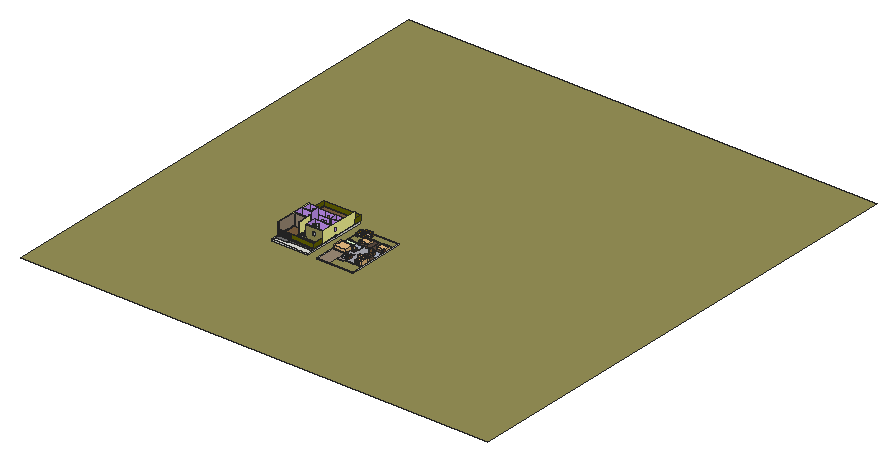
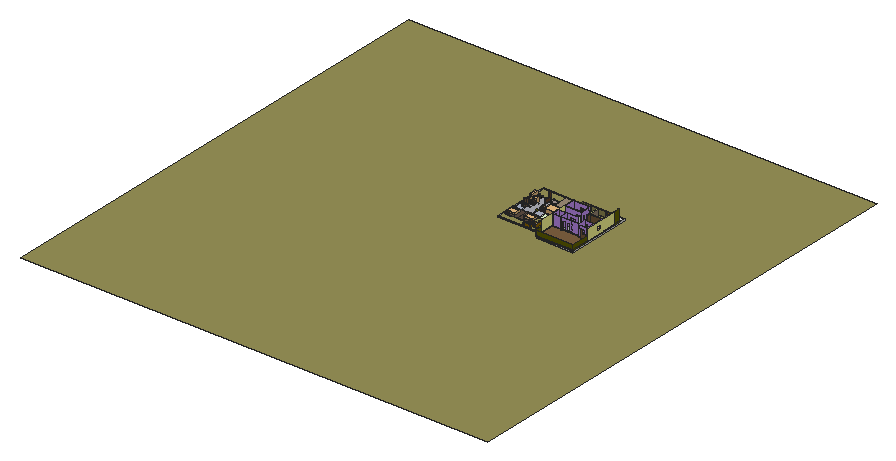
# SketchUp Ruby script. Lengths in inches.
U = 1.inch
M = Sketchup.active_model
def pt(a) = Geom::Point3d.new(a.map { |v| v * U })
def face(e, loops, mat)
  f = e.add_face(loops[0].map { |a| pt(a) })
  loops[1..].each { |l| e.add_face(l.map { |a| pt(a) }).erase! }
  f.material = f.back_material = mat if mat
  f
end
# faces: each face lists its corners as indices into pts; further lists are holes
def faces(e, pts, list, mat = nil) = list.each { |f| face(e, (f[0].is_a?(Array) ? f : [f]).map { |l| l.map { |i| pts[i] } }, mat) }
# xy, xz, yz: faces in a plane at the given z, y or x. An outline is a flat list of corners, or four numbers for a rectangle; further outlines are holes
def ring(l) = l.size == 4 ? [[l[0], l[1]], [l[2], l[1]], [l[2], l[3]], [l[0], l[3]]] : l.each_slice(2).to_a
def flat(e, list, mat, &to3) = list.each { |f| face(e, (f[0].is_a?(Array) ? f : [f]).map { |l| ring(l).map { |u, v| to3.(u, v) } }, mat) }
def xy(e, z, list, mat = nil) = flat(e, list, mat) { |x, y| [x, y, z] }
def xz(e, y, list, mat = nil) = flat(e, list, mat) { |x, z| [x, y, z] }
def yz(e, x, list, mat = nil) = flat(e, list, mat) { |y, z| [x, y, z] }
def lines(e, pts, list) = list.each { |a, b| e.add_line(pt(pts[a]), pt(pts[b])) }
# prism: a flat outline (further loops are holes) pulled along v
def prism(e, loops, v, mat = nil)
  f = face(e, loops, mat); d = Geom::Vector3d.new(v.map { |x| x * U })
  f.pushpull(f.normal.samedirection?(d) ? d.length : -d.length)
end
def box(e, o, s, mat = nil) = prism(e, [[o, [o[0] + s[0], o[1], o[2]], [o[0] + s[0], o[1] + s[1], o[2]], [o[0], o[1] + s[1], o[2]]]], [0, 0, s[2]], mat)
def at(x, y, z, deg = 0) = Geom::Transformation.translation(pt([x, y, z])) * Geom::Transformation.rotation(ORIGIN, Z_AXIS, deg.degrees)
def axes(o, x, y, z) = Geom::Transformation.new([*x, 0, *y, 0, *z, 0, *pt(o).to_a, 1])
def part(name) = M.definitions.add(name)
# library, detail: a bought-in or finely detailed component or shape, given as its bounding box
def library(name, o, s) = part(name).tap { |d| box(d.entities, o, s) }
def detail(e, o, s) = box(e.add_group.entities, o, s)
def put(e, d, t, mat = nil) = e.add_instance(d, t).tap { |i| i.material = mat if mat }
def group(e, t, mat = nil) = e.add_group.tap { |g| g.transformation = t; g.material = mat if mat }.entities
root = M.entities
M.materials.add("C01_Vanilla_Cream").color = [255, 230, 206]
M.materials.add("D07_Ochre_Flame").color = [153, 107, 0]
M.materials.add("E01_Mint_Frost").color = [255, 255, 204]
M.materials.add("E02_Pale_Lime").color = [255, 255, 153]
M.materials.add("E08_Lime_Depth").color = [102, 102, 0]
M.materials.add("Glass_Sky Reflection_01").color = [126, 138, 183]
M.materials["Glass_Sky Reflection_01"].alpha = 0.25
M.materials.add("J02_Lavender_Veil").color = [204, 153, 255]
M.materials.add("M05_Graphite_Haze").color = [114, 114, 114]
M.materials.add("M09_Shadow_Night").color = [0, 0, 0]
M.materials.add("Marble_01_1K").color = [230, 255, 211]
M.materials.add("Marble_03_1K").color = [175, 182, 201]
M.materials.add("Marble_06_1K").color = [165, 150, 147]
M.materials.add("Marble_07_1K").color = [36, 34, 36]
M.materials.add("Marble_20_1K").color = [172, 173, 182]
M.materials.add("Metal_06_1K").color = [238, 236, 231]
M.materials.add("Plaster_02_1K").color = [157, 140, 119]
M.materials.add("Plywood_01_1K").color = [125, 96, 64]
M.materials.add("Soil_04_1K").color = [152, 146, 88]
M.materials.add("Wood_Floor_01_1K").color = [146, 111, 76]
M.materials.add("Wood_Floor_12_1K").color = [92, 75, 65]
M.materials.add("Wood_Veneer_15_1K").color = [103, 69, 45]
c1 = library("Group\#68",[0,0,0],[137.375,104.9375,36.125])
c2 = library("Group\#24",[0,0,0],[4.375,4.375,0.1875])
c3 = part("Group\#9")
box(c3.entities,[0,0,0],[0.75,3.75,0.1875],"Metal_06_1K")
c4 = part("Group\#2")
xy(c4.entities,0,[[0,-16.81,18.0625,0],[0,0,18.0625,55.25]],"Wood_Veneer_15_1K")
xy(c4.entities,36,[[0,0,18.0625,55.25]],"Wood_Veneer_15_1K")
xy(c4.entities,84,[[0,-16.81,18.0625,0]],"Wood_Veneer_15_1K")
xz(c4.entities,-16.81,[[0,0,18.0625,84]],"Wood_Veneer_15_1K")
xz(c4.entities,0,[[0,0,18.0625,36],[0,36,18.0625,84]],"Wood_Veneer_15_1K")
xz(c4.entities,55.25,[[0,0,18.0625,36]],"Wood_Veneer_15_1K")
yz(c4.entities,0,[[-16.81,0,0,84],[0,0,55.25,36]],"Wood_Veneer_15_1K")
yz(c4.entities,18.0625,[[[-16.81,0,0,84],[-14.81,2,-2,82]],[0,0,27.625,27.91],[27.625,0,55.25,27.91],[-14.81,2,-2,35],[0,27.91,55.25,36],
  [-14.81,35,-2,36],[-14.81,36,-2,50.3125],[-14.81,50.3125,-2,51.3125],[-14.81,51.3125,-2,65.85],[-14.81,65.85,-2,66.85],
  [-14.81,66.85,-2,82]],"Wood_Veneer_15_1K")
g1 = group(c4.entities,at(18.0625,23.18,16.77))
box(g1,[0,0,0],[0.2,1.5,6.25],"Metal_06_1K")
g2 = group(c4.entities,at(18.0625,29.74,16.77))
box(g2,[0,0,0],[0.2,1.5,6.25],"Metal_06_1K")
put(c4.entities,c3,axes([18.0625,-4.49,72.03],[0,1,0],[0,0,1],[1,0,0]))
put(c4.entities,c3,axes([18.0625,-4.49,57.4],[0,1,0],[0,0,1],[1,0,0]))
put(c4.entities,c3,axes([18.0625,-4.49,42.9],[0,1,0],[0,0,1],[1,0,0]))
put(c4.entities,c3,axes([18.0625,-4.49,20.71],[0,1,0],[0,0,1],[1,0,0]))
c5 = part("Group\#41")
xy(c5.entities,0,[[[0,0,32.5625,34],[3.65,3.65,28.91,30.35]]],"D07_Ochre_Flame")
xy(c5.entities,18.3125,[[[0,0,32.5625,34],[3.65,3.65,28.91,30.35]]],"D07_Ochre_Flame")
xy(c5.entities,18.3125,[[3.65,3.65,28.91,30.35]],"Plaster_02_1K")
xz(c5.entities,0,[[0,0,32.5625,18.3125]],"D07_Ochre_Flame")
xz(c5.entities,3.65,[[3.65,0,28.91,18.3125]],"D07_Ochre_Flame")
xz(c5.entities,30.35,[[3.65,0,28.91,18.3125]],"D07_Ochre_Flame")
xz(c5.entities,34,[[0,0,32.5625,18.3125]],"D07_Ochre_Flame")
yz(c5.entities,0,[[0,0,34,18.3125]],"D07_Ochre_Flame")
yz(c5.entities,3.65,[[3.65,0,30.35,18.3125]],"D07_Ochre_Flame")
yz(c5.entities,28.91,[[3.65,0,30.35,18.3125]],"D07_Ochre_Flame")
yz(c5.entities,32.5625,[[0,0,34,18.3125]],"D07_Ochre_Flame")
c6 = library("Group\#27",[0,0,0],[94.3125,62.5,20])
c7 = part("Group\#17")
box(c7.entities,[0,0,0],[4,4,24])
c8 = part("Group\#16")
box(c8.entities,[0,0,0],[4,4,24])
c9 = part("Group\#29")
box(c9.entities,[0,0,0],[20.5,20.5,18],"Wood_Veneer_15_1K")
c10 = part("Group\#12")
detail(c10.entities,[-3,0,0],[54,27,43.625])
c11 = part("Group\#11")
detail(c11.entities,[0,0,0],[24,24,25.375])
c12 = part("Group\#10")
detail(c12.entities,[0,-4,0],[28,80,43.625])
c13 = part("Group\#14")
box(c13.entities,[0,0,0],[4,4,24])
c14 = part("Group\#15")
box(c14.entities,[0,0,0],[4,4,24])
c15 = part("Group\#38")
xy(c15.entities,0,[[67.3125,0,69.625,27.1875],[-2.33,24.1875,67.3125,27.1875]],"D07_Ochre_Flame")
xy(c15.entities,18.3125,[[0,0,22.82,24.1875],[22.82,0,45.07,24.1875],[45.07,0,67.3125,24.1875]],"C01_Vanilla_Cream")
xy(c15.entities,24.5625,[[67.3125,0,69.625,27.1875]],"D07_Ochre_Flame")
xy(c15.entities,28.6875,[[-2.33,0,0,24.1875]],"D07_Ochre_Flame")
xy(c15.entities,33.375,[[-2.33,24.1875,67.3125,27.1875]],"D07_Ochre_Flame")
xz(c15.entities,0,[[0,0,22.82,18.3125],[22.82,0,45.07,18.3125],[45.07,0,67.3125,18.3125]],"C01_Vanilla_Cream")
xz(c15.entities,0,[[-2.33,0,0,28.6875],[67.3125,0,69.625,24.5625]],"D07_Ochre_Flame")
xz(c15.entities,24.1875,[[-2.33,0,67.3125,0,67.3125,18.3125,0,18.3125,0,28.6875,-2.33,28.6875],[0,18.3125,22.82,33.375],[22.82,18.3125,45.07,33.375],[45.07,18.3125,67.3125,33.375],[-2.33,28.6875,0,33.375]],"D07_Ochre_Flame")
xz(c15.entities,27.1875,[[-2.33,0,67.3125,33.375],[67.3125,0,69.625,24.5625]],"D07_Ochre_Flame")
yz(c15.entities,-2.33,[[0,0,24.1875,28.6875],[24.1875,0,27.1875,33.375]],"D07_Ochre_Flame")
yz(c15.entities,0,[[0,18.3125,24.1875,28.6875]],"D07_Ochre_Flame")
yz(c15.entities,67.3125,[[0,0,24.1875,18.3125],[0,18.3125,24.1875,24.5625]],"C01_Vanilla_Cream")
yz(c15.entities,67.3125,[[24.1875,0,27.1875,24.5625],[24.1875,24.5625,27.1875,33.375]],"D07_Ochre_Flame")
yz(c15.entities,69.625,[[0,0,27.1875,24.5625]],"D07_Ochre_Flame")
c16 = part("Group\#43")
box(c16.entities,[0,0,0],[1,4.5625,0.25],"Metal_06_1K")
c17 = part("Group\#42")
xy(c17.entities,0,[[0,-1.93,40.35,0],[0,0,40.35,21.25]],"Plywood_01_1K")
xy(c17.entities,25.125,[[0,0,40.35,21.25]],"Marble_07_1K")
xy(c17.entities,25.1875,[[20.85,8.75,21.39,8.86,21.89,9.11,22.3,9.47,22.61,9.94,22.79,10.46,22.82,11.01,22.71,11.56,22.47,12.06,22.1,12.47,21.64,12.78,21.11,12.96,20.56,12.99,20.01,12.88,19.52,12.63,19.1,12.27,18.79,11.81,18.62,11.28,18.58,10.73,18.69,10.18,18.9375,9.69,19.31,9.27,19.77,8.96,20.29,8.79]],"M09_Shadow_Night")
xy(c17.entities,25.1875,[[[8.8,4,31.8,17.68],[20.85,8.75,20.29,8.79,19.77,8.96,19.31,9.27,18.9375,9.69,18.69,10.18,18.58,10.73,18.62,11.28,18.79,11.81,19.1,12.27,19.52,12.63,20.01,12.88,20.56,12.99,21.11,12.96,21.64,12.78,22.1,12.47,22.47,12.06,22.71,11.56,22.82,11.01,22.79,10.46,22.61,9.94,22.3,9.47,21.89,9.11,21.39,8.86]]],"Marble_07_1K")
xy(c17.entities,26,[[0,-1.93,40.35,0]],"Plywood_01_1K")
xy(c17.entities,26.5625,[[[0,0,40.35,21.25],[8.8,4,31.8,17.68]]],"Marble_07_1K")
xy(c17.entities,71.66,[[0,-1.93,40.35,0]],"Plywood_01_1K")
xz(c17.entities,-1.93,[[0,0,40.35,26],[0,26,40.35,71.66]],"Plywood_01_1K")
xz(c17.entities,0,[[0,25.125,40.35,26],[0,26,40.35,26.5625]],"Marble_07_1K")
xz(c17.entities,0,[[0,0,40.35,25.125],[0,26.5625,40.35,71.66]],"Plywood_01_1K")
xz(c17.entities,4,[[8.8,25.1875,31.8,26.5625]],"Marble_07_1K")
xz(c17.entities,17.68,[[8.8,25.1875,31.8,26.5625]],"Marble_07_1K")
xz(c17.entities,21.25,[[0,25.125,40.35,26.5625]],"Marble_07_1K")
xz(c17.entities,21.25,[[0,0,20.17,21],[20.17,0,40.35,21],[0,21,40.35,25.125]],"Plywood_01_1K")
yz(c17.entities,0,[[0,25.125,21.25,26.5625]],"Marble_07_1K")
yz(c17.entities,0,[[-1.93,0,0,26],[0,0,21.25,25.125],[-1.93,26,0,71.66]],"Plywood_01_1K")
yz(c17.entities,8.8,[[4,25.1875,17.68,26.5625]],"Marble_07_1K")
yz(c17.entities,31.8,[[4,25.1875,17.68,26.5625]],"Marble_07_1K")
yz(c17.entities,40.35,[[0,25.125,21.25,26.5625]],"Marble_07_1K")
yz(c17.entities,40.35,[[-1.93,0,0,26],[0,0,21.25,25.125],[-1.93,26,0,71.66]],"Plywood_01_1K")
put(c17.entities,c16,axes([22.63,21.25,13.17],[-1,0,0],[0,0,1],[0,1,0]))
put(c17.entities,c16,axes([18.69,21.25,13.17],[-1,0,0],[0,0,1],[0,1,0]))
put(c17.entities,c16,axes([22.61,21.25,24.2],[0,0,-1],[-1,0,0],[0,1,0]))
c18 = part("Group\#40")
box(c18.entities,[0,4,0],[19.9375,19.25,18.3125],"D07_Ochre_Flame")
c19 = library("Group\#36",[0,0,0],[17.25,17.25,38])
c20 = part("Group\#70")
box(c20.entities,[0,0,0],[9,39,6],"Wood_Floor_12_1K")
c21 = library("Group\#28",[0,0,0],[94.3125,62.5,20])
c22 = library("Group\#18",[0,0,-13],[137.375,104.9375,49.125])
c23 = part("Group\#13")
detail(c23.entities,[-5.9375,-5.9375,0],[39.25,56.8125,1])
c24 = part("Group\#48")
xy(c24.entities,0,[[0,0,73.6875,17.1875]],"Marble_06_1K")
xy(root,0,[[0,0,5379.41,5576.625]],"Soil_04_1K")
xy(root,18,[[1567.04,1740.42,1567.04,2402.64,1987.04,2401.71,1987.04,1740.42,1982.36,1740.42,1982.36,1862.58,1788.11,1862.58,1788.11,1845.39,1714.42,1845.39,1714.42,1862.58,1713.42,1862.58,1713.42,1967.64,1576.04,1967.64,1576.04,1740.42],[1576.04,1740.42,1576.04,1967.64,1713.42,1967.64,1713.42,1862.58,1714.42,1862.58,1714.42,1740.42]],"Plywood_01_1K")
xy(root,18,[[1714.42,1740.42,1714.42,1845.39,1788.11,1845.39,1788.11,1862.58,1982.36,1862.58,1982.36,1740.42]],"Soil_04_1K")
xy(root,22.48,[[1714.42,1740.42,1982.36,1745.11]],"Soil_04_1K")
xy(root,24,[[1600.04,2000.64,1713.42,2000.64,1713.42,2030.95,1675.875,2030.95,1675.875,2081.58,1642.13,2081.58,1642.13,2057.58,1600.04,2057.58],[1576.04,2087.58,1678.04,2183.58]],"Marble_01_1K")
xy(root,24,[[1684.04,2081.58,1768.04,2171.58],[1894.04,2087.58,1978.04,2171.58]],"Marble_03_1K")
xy(root,24,[[[1794.11,1871.58,1978.04,1871.58,1978.04,1991.58,1840.09,1991.58,1840.09,1997.58,1861.04,1997.58,1861.04,2038.58,1940.04,2038.58,1940.04,2040.58,1888.04,2040.58,1888.04,2171.58,1768.04,2171.58,1768.04,2081.58,1675.875,2081.58,1675.875,2030.95,1713.42,2030.95,1713.42,2000.64,1722.42,2000.64,1722.42,1901.49,1788.11,1901.49,1788.11,1951.47,1794.11,1951.47],[1788.11,1985.89,1788.11,1997.58,1798.45,1997.58,1798.45,1991.58,1794.11,1991.58,1794.11,1985.89]]],"Marble_20_1K")
xy(root,24,[[1567.04,1740.42,1576.04,2005.11],[1567.04,2005.11,1567.04,2402.64,1987.04,2401.71,1987.04,2015.58,1978.04,2015.58,1978.04,2171.58,1684.04,2171.58,1684.04,2087.58,1678.04,2087.58,1678.04,2183.58,1576.04,2183.58,1576.04,2005.11],[1987.04,2401.71,1567.04,2402.64,1987.04,2402.64]],"Plywood_01_1K")
xy(root,30,[[1567.04,1814.64,1576.04,1814.64,1576.04,2087.58,1684.04,2087.58,1684.04,2171.58,1978.04,2171.58,1978.04,2015.58,1987.04,2015.58,1987.04,2402.64,1567.04,2402.64]],"Plywood_01_1K")
xz(root,1740.42,[[1567.04,18,1576.04,24],[1714.42,18,1982.36,22.48],[1982.36,18,1987.04,24],[1714.42,22.48,1982.36,24],[1567.04,24,1576.04,156],
  [1714.42,24,1987.04,30],[1714.42,30,1987.04,84]],"E08_Lime_Depth")
xz(root,1740.42,[[1576.04,18,1714.42,24]],"Plywood_01_1K")
xz(root,1745.11,[[1714.42,22.48,1982.36,84]],"Soil_04_1K")
xz(root,1845.39,[[1714.42,18,1788.11,30]],"Soil_04_1K")
xz(root,1862.58,[[1714.42,30,1788.11,30,1788.11,36,1722.42,36,1722.42,36.4375,1714.42,36.4375]],"Marble_06_1K")
xz(root,1862.58,[[1713.42,18,1714.42,30],[1713.42,30,1714.42,156]],"Plywood_01_1K")
xz(root,1862.58,[[[1788.11,18,1788.11,156,1978.04,156,1978.04,84,1982.36,84,1982.36,18],[1862.07,72,1910.07,120]]],"Soil_04_1K")
xz(root,1871.58,[[[1794.11,24,1978.04,156],[1862.07,72,1910.07,120]]],"J02_Lavender_Veil")
xz(root,1901.49,[[1722.42,24,1788.11,36]],"Marble_20_1K")
xz(root,1940.04,[[1717.92,24,1722.42,36]],"Plywood_01_1K")
xz(root,1951.47,[[1788.11,24,1794.11,120]],"J02_Lavender_Veil")
xz(root,1967.64,[[1576.04,18,1713.42,156]],"Plaster_02_1K")
xz(root,1976.64,[[1576.04,24,1713.42,156]],"Plywood_01_1K")
xz(root,1985.89,[[1788.11,24,1794.11,120]],"J02_Lavender_Veil")
xz(root,1991.58,[[1794.11,24,1798.45,24,1798.45,120,1840.09,120,1840.09,24,1978.04,24,1978.04,156,1794.11,156]],"J02_Lavender_Veil")
xz(root,1997.58,[[1788.11,24,1788.11,156,1978.04,156,1978.04,36,1861.04,36,1861.04,24,1840.09,24,1840.09,120,1798.45,120,1798.45,24]],"J02_Lavender_Veil")
xz(root,1997.58,[[1861.04,24,1870.04,36],[1870.04,24,1879.04,36],[1879.04,24,1888.04,36],[1888.04,24,1897.04,36],[1897.04,24,1906.04,36],
  [1906.04,24,1915.04,36],[1915.04,24,1924.04,36],[1924.04,24,1933.04,36],[1933.04,24,1942.04,36],[1942.04,24,1978.04,36]],"Plywood_01_1K")
xz(root,2000.64,[[1713.42,24,1721.79,156],[1721.79,24,1722.42,156]],"J02_Lavender_Veil")
xz(root,2000.64,[[1600.04,24,1713.42,37]],"Wood_Veneer_15_1K")
xz(root,2005.11,[[1571.54,24,1576.04,66]],"Plywood_01_1K")
xz(root,2015.58,[[1978.04,24,1982.54,30],[1982.54,24,1987.04,30],[1978.04,30,1982.54,36],[1982.54,30,1987.04,36]],"Plywood_01_1K")
xz(root,2038.58,[[1861.04,24,1940.04,36]],"Marble_20_1K")
xz(root,2040.58,[[1888.04,24,1940.04,36]],"Marble_20_1K")
xz(root,2057.58,[[1600.04,24,1642.13,37]],"Wood_Veneer_15_1K")
xz(root,2081.58,[[1642.13,24,1644.54,24,1644.54,120,1675.875,120,1675.875,24,1684.04,24,1684.04,156,1576.04,156,1576.04,37,1642.13,37],[1768.04,24,1768.04,156,1888.04,156,1888.04,24,1861.04,24,1861.04,120,1794.48,120,1794.48,24]],"J02_Lavender_Veil")
xz(root,2081.58,[[1644.54,24,1675.875,36]],"Marble_01_1K")
xz(root,2087.58,[[1576.04,24,1644.54,30],[1675.875,24,1678.04,30],[1894.04,24,1978.04,156],[1576.04,30,1576.04,156,1678.04,156,1678.04,30,1675.875,30,1675.875,120,1644.54,120,1644.54,30]],"J02_Lavender_Veil")
xz(root,2087.58,[[1644.54,24,1675.875,30],[1644.54,30,1675.875,36]],"Marble_01_1K")
xz(root,2087.58,[[1678.04,24,1684.04,30]],"Plywood_01_1K")
xz(root,2171.58,[[1684.04,24,1768.04,30],[1768.04,24,1788.97,30],[1824.97,24,1837.82,30],[1873.82,24,1888.04,30],[1894.04,24,1978.04,30],
  [1684.04,30,1768.04,156],[1768.04,30,1788.97,30,1788.97,120,1824.97,120,1824.97,30,1837.82,30,1837.82,120,1873.82,120,1873.82,30,1888.04,30,1888.04,156,1768.04,156],[1894.04,30,1978.04,156]],"J02_Lavender_Veil")
xz(root,2171.58,[[1788.97,24,1824.97,30],[1837.82,24,1873.82,30],[1788.97,30,1824.97,36],[1837.82,30,1873.82,36]],"Marble_20_1K")
xz(root,2171.58,[[1888.04,24,1894.04,30]],"Plywood_01_1K")
xz(root,2183.58,[[1576.04,24,1605.14,24,1605.14,120,1641.14,120,1641.14,120.0625,1644.54,120.0625,1644.54,120,1675.875,120,1675.875,24,1678.04,24,1678.04,156,1576.04,156]],"J02_Lavender_Veil")
xz(root,2183.58,[[1644.54,24,1675.875,36]],"Marble_01_1K")
xz(root,2183.58,[[1605.14,24,1644.54,24,1644.54,120,1641.14,120,1641.14,72,1605.14,72]],"Plywood_01_1K")
xz(root,2402.64,[[1567.04,24,1987.04,30],[1567.04,30,1987.04,84]],"E08_Lime_Depth")
yz(root,1567.04,[[[1814.64,30,2192.58,156],[2005.11,66,2053.11,114]]],"E02_Pale_Lime")
yz(root,1567.04,[[1740.42,18,2402.64,24],[1740.42,24,1814.64,30],[1814.64,24,2005.11,30],[2005.11,24,2402.64,30],[1740.42,30,1814.64,156],
  [2192.58,30,2402.64,84]],"E08_Lime_Depth")
yz(root,1576.04,[[1740.42,30,1749.42,156]],"E08_Lime_Depth")
yz(root,1576.04,[[1976.64,24,2005.11,30],[2087.58,24,2183.58,156],[1976.64,30,2005.11,30,2005.11,114,2053.11,114,2053.11,37,2081.58,37,2081.58,156,1976.64,156]],"J02_Lavender_Veil")
yz(root,1576.04,[[1740.42,18,1967.64,24],[1749.42,24,1967.64,30],[1749.42,30,1967.64,156]],"Plaster_02_1K")
yz(root,1576.04,[[1740.42,24,1749.42,30],[1967.64,24,1976.64,30],[2005.11,24,2087.58,30]],"Plywood_01_1K")
yz(root,1600.04,[[2000.64,24,2057.58,37]],"Wood_Veneer_15_1K")
yz(root,1642.13,[[2057.58,24,2081.58,37]],"Wood_Veneer_15_1K")
yz(root,1678.04,[[2087.58,24,2087.58,156,2183.58,156,2183.58,24,2141.58,24,2141.58,37.9375,2117.58,37.9375,2117.58,24]],"J02_Lavender_Veil")
yz(root,1678.04,[[2117.58,24,2141.58,37.9375]],"Plywood_01_1K")
yz(root,1684.04,[[2081.58,24,2087.58,24,2087.58,30,2117.58,30,2117.58,37.9375,2141.58,37.9375,2141.58,30,2171.58,30,2171.58,156,2081.58,156],[2087.58,24,2117.58,30],[2141.58,24,2171.58,30]],"J02_Lavender_Veil")
yz(root,1684.04,[[2117.58,24,2141.58,30],[2117.58,30,2141.58,37.9375]],"Plywood_01_1K")
yz(root,1713.42,[[[1862.58,18,1967.64,156],[1916.04,36,1940.04,108]]],"Plaster_02_1K")
yz(root,1713.42,[[1976.64,24,2000.64,156]],"Plywood_01_1K")
yz(root,1714.42,[[1845.39,18,1862.58,30],[1740.42,24,1745.11,84]],"Plywood_01_1K")
yz(root,1714.42,[[1740.42,22.48,1745.11,24]],"Soil_04_1K")
yz(root,1722.42,[[1901.49,24,1916.04,24,1916.04,108,1940.04,108,1940.04,24,2000.64,24,2000.64,156,1912.1875,156,1912.1875,135.24,1900.1875,135.24,1900.1875,156,1862.58,156,1862.58,36,1901.49,36]],"E02_Pale_Lime")
yz(root,1722.42,[[1916.04,24,1940.04,36]],"Marble_20_1K")
yz(root,1788.11,[[1901.49,24,1901.49,135.24,1912.1875,135.24,1912.1875,156,1997.58,156,1997.58,24,1985.89,24,1985.89,120,1951.47,120,1951.47,24]],"J02_Lavender_Veil")
yz(root,1788.11,[[1845.39,18,1862.58,30]],"Soil_04_1K")
yz(root,1794.11,[[1871.58,24,1951.47,24,1951.47,120,1985.89,120,1985.89,24,1991.58,24,1991.58,156,1871.58,156]],"J02_Lavender_Veil")
yz(root,1798.45,[[1991.58,24,1997.58,120]],"J02_Lavender_Veil")
yz(root,1840.09,[[1991.58,24,1997.58,120]],"J02_Lavender_Veil")
yz(root,1861.04,[[1997.58,24,2036.58,36],[2036.58,24,2038.58,36]],"Marble_20_1K")
yz(root,1888.04,[[2081.58,24,2081.58,156,2171.58,156,2171.58,24,2167.61,24,2167.61,120,2137.61,120,2137.61,24]],"J02_Lavender_Veil")
yz(root,1888.04,[[2040.58,24,2042.58,36],[2042.58,24,2081.58,36],[2137.61,24,2167.61,36]],"Marble_20_1K")
yz(root,1894.04,[[2087.58,24,2137.61,24,2137.61,120,2167.61,120,2167.61,24,2171.58,24,2171.58,156,2087.58,156]],"J02_Lavender_Veil")
yz(root,1894.04,[[2137.61,24,2167.61,36]],"Marble_03_1K")
yz(root,1910.07,[[1867.08,24,1871.58,36]],"Plywood_01_1K")
yz(root,1940.04,[[2038.58,24,2040.58,36]],"Marble_20_1K")
yz(root,1978.04,[[1871.58,24,1991.58,156],[2087.58,24,2171.58,30],[[2087.58,30,2171.58,156],[2117.58,120.9375,2141.58,144.9375]]],"J02_Lavender_Veil")
yz(root,1978.04,[[1997.58,24,2015.58,36],[2015.58,24,2087.58,30]],"Plywood_01_1K")
yz(root,1982.36,[[1740.42,18,1862.58,18,1862.58,84,1745.11,84,1745.11,22.48,1740.42,22.48]],"Soil_04_1K")
yz(root,1987.04,[[[1862.58,30,2015.58,30,2015.58,36,2063.58,36,2063.58,30,2318.58,30,2318.58,156,1862.58,156],[2015.58,72,2063.58,120.04],[2117.58,120.9375,2141.58,144.9375]],[2015.58,30,2063.58,36]],"E02_Pale_Lime")
yz(root,1987.04,[[1740.42,18,2401.71,24],[1740.42,24,1814.64,30],[1814.64,24,2015.58,30],[2015.58,24,2402.64,30],[1740.42,30,1862.58,84],
  [2318.58,30,2402.64,84]],"E08_Lime_Depth")
p = [[1567.04,2402.64,24],[1987.04,2401.71,24],[1987.04,2401.71,18],[1567.04,2402.64,18],[2197.13,2047.35,6],[2197.13,2049.35,6],
  [1978.04,2063.58,30],[1978.04,2063.58,36],[1987.04,1814.64,30],[1978.04,1814.64,30]]
faces(root,p,[[0,1,2,3]],"E08_Lime_Depth")
lines(root,p,[[4,5],[6,7],[8,9]])
g3 = group(root,at(2086.13,1724.92,0))
xy(g3,0,[[0,0,420,588]])
xy(g3,6,[[295.03,47.9375,343.03,52.4375],[295.03,52.4375,343.03,56.9375],[196.74,80.85,208.74,83.85],[196.74,83.85,208.74,86.85],[146.375,101.4,150.875,125.4],
  [150.875,101.4,155.375,125.4],[0,190.47,4.5,238.47],[4.5,190.47,9,238.47],[411,200.9375,415.5,248.9375],[415.5,200.9375,420,248.9375],
  [111,302.9375,114,326.9375],[114,302.9375,117,326.9375],[411,302.9375,415.5,326.9375],[415.5,302.9375,420,326.9375],[38.09,368.9375,74.09,373.4375],
  [74.09,368.9375,77.5,377.9375],[77.5,368.9375,108.83,377.9375],[38.09,373.4375,74.09,377.9375],[165,494.9375,213,499.4375],[315,494.9375,363,499.4375],
  [165,499.4375,213,503.9375],[315,499.4375,363,503.9375]])
xy(g3,6,[[0,-74.22,0,190.47,9,190.47,9,162,146.375,162,146.375,186,155.375,186,155.375,125.4,146.375,125.4,146.375,153,9,153,9,-65.22,411,-65.22,411,47.9375,343.03,47.9375,343.03,56.9375,411,56.9375,411,176.9375,273.05,176.9375,273.05,182.9375,411,182.9375,411,200.9375,420,200.9375,420,-74.22],[146.375,47.9375,155.375,47.9375,155.375,80.85,160.74,80.85,160.74,86.85,155.375,86.85,155.375,101.4,146.375,101.4],[221.0625,47.9375,295.03,47.9375,295.03,56.9375,227.0625,56.9375,227.0625,136.83,221.0625,136.83,221.0625,86.85,208.74,86.85,208.74,80.85,221.0625,80.85],[221.0625,171.25,227.0625,171.25,227.0625,176.9375,231.41,176.9375,231.41,182.9375,221.0625,182.9375],[0,238.47,9,238.47,9,266.9375,77.5,266.9375,77.5,272.9375,9,272.9375,9,368.9375,38.09,368.9375,38.09,377.9375,9,377.9375,9,579,411,579,411,503.9375,363,503.9375,363,494.9375,411,494.9375,411,362.9375,306.78,362.9375,306.78,356.9375,321,356.9375,321,352.97,327,352.97,327,356.9375,411,356.9375,411,326.9375,420,326.9375,420,588,0,588],
  [411,248.9375,420,248.9375,420,302.9375,411,302.9375,411,272.9375,327,272.9375,327,322.97,321,322.97,321,272.9375,294,272.9375,294,266.9375,411,266.9375],[108.83,266.9375,227.4375,266.9375,227.4375,272.9375,207,272.9375,207,322.97,201,322.97,201,272.9375,117,272.9375,117,302.9375,111,302.9375,111,272.9375,108.83,272.9375],[111,326.9375,117,326.9375,117,356.9375,201,356.9375,201,352.97,207,352.97,207,356.9375,221.92,356.9375,221.92,362.9375,117,362.9375,117,494.9375,165,494.9375,165,503.9375,111,503.9375,111,377.9375,108.83,377.9375,108.83,368.9375,111,368.9375],[257.92,356.9375,270.78,356.9375,270.78,362.9375,267,362.9375,267,494.9375,315,494.9375,315,503.9375,213,503.9375,213,494.9375,261,494.9375,261,362.9375,257.92,362.9375]],"E08_Lime_Depth")
xy(g3,6,[[33,186,146.375,186,146.375,216.3125,108.83,216.3125,108.83,266.9375,75.09,266.9375,75.09,242.9375,33,242.9375],[77.5,266.9375,108.83,272.9375],[9,272.9375,111,368.9375]],"Marble_01_1K")
xy(g3,6,[[117,272.9375,201,356.9375],[327,272.9375,411,356.9375],[201,322.97,207,352.97],[321,322.97,327,352.97]],"Marble_03_1K")
xy(g3,6,[[147.375,30.75,221.0625,30.75,221.0625,38.75,155.375,38.75,155.375,47.9375,147.375,47.9375],[155.375,38.75,221.0625,80.85]],"Marble_06_1K")
xy(g3,6,[[[227.0625,56.9375,411,56.9375,411,176.9375,273.05,176.9375,273.05,182.9375,294,182.9375,294,223.9375,373,223.9375,373,225.9375,321,225.9375,321,266.9375,294,266.9375,294,272.9375,321,272.9375,321,356.9375,207,356.9375,207,272.9375,227.4375,272.9375,227.4375,266.9375,108.83,266.9375,108.83,216.3125,146.375,216.3125,146.375,186,155.375,186,155.375,86.85,221.0625,86.85,221.0625,136.83,227.0625,136.83],[221.0625,171.25,221.0625,182.9375,231.41,182.9375,231.41,176.9375,227.0625,176.9375,227.0625,171.25]],[160.74,80.85,196.74,86.85]],"Marble_20_1K")
xy(g3,6,[[294,221.9375,375,221.9375,375,227.9375,321,227.9375,321,225.9375,373,225.9375,373,223.9375,294,223.9375]],"Metal_06_1K")
xy(g3,6,[[9,-65.22,9,153,146.375,153,146.375,47.9375,147.375,47.9375,147.375,-65.22]],"Plaster_02_1K")
xy(g3,6,[[147.375,-65.22,411,-65.22,411,47.9375,221.0625,47.9375,221.0625,30.75,147.375,30.75],[9,377.9375,111,377.9375,111,503.9375,411,503.9375,411,579,9,579]],"Soil_04_1K")
xy(g3,6,[[294,182.9375,303,221.9375],[303,182.9375,312,221.9375],[312,182.9375,321,221.9375],[321,182.9375,330,221.9375],[330,182.9375,339,221.9375],
  [339,182.9375,348,221.9375],[348,182.9375,357,221.9375],[357,182.9375,366,221.9375],[366,182.9375,375,221.9375],[375,182.9375,411,266.9375],
  [321,227.9375,330,266.9375],[330,227.9375,339,266.9375],[339,227.9375,348,266.9375],[348,227.9375,357,266.9375],[357,227.9375,366,266.9375],
  [366,227.9375,375,266.9375],[117,362.9375,261,494.9375],[267,362.9375,411,494.9375]],"Wood_Floor_12_1K")
xy(g3,6,[[221.92,356.9375,257.92,362.9375],[270.78,356.9375,306.78,362.9375]],"Wood_Veneer_15_1K")
xy(g3,43,[[12.47,221.72,30.47,222.35]],"Metal_06_1K")
xz(g3,-74.22,[[0,0,420,6]])
xz(g3,162,[[9,6,146.375,7]],"Wood_Veneer_15_1K")
xz(g3,186,[[33,6,146.375,7]],"Wood_Veneer_15_1K")
xz(g3,242.9375,[[33,6,75.09,7]],"Wood_Veneer_15_1K")
xz(g3,266.9375,[[9,6,75.09,7]],"Wood_Veneer_15_1K")
xz(g3,588,[[0,0,420,6]])
yz(g3,0,[[-74.22,0,0,6],[0,0,588,6]])
yz(g3,9,[[162,6,190.47,7],[190.47,6,238.47,7],[238.47,6,266.9375,7]],"Wood_Veneer_15_1K")
yz(g3,33,[[186,6,242.9375,7]],"Wood_Veneer_15_1K")
yz(g3,75.09,[[242.9375,6,266.9375,7]],"Wood_Veneer_15_1K")
yz(g3,146.375,[[162,6,186,7]],"Wood_Veneer_15_1K")
yz(g3,420,[[-74.22,0,0,6],[0,0,588,6]])
p = [[411,0,0],[411,0,6],[9,0,0],[9,0,6]]
lines(g3,p,[[0,1],[2,3]])
put(g3,c1,at(9,162,7))
put(g3,c2,at(20.51,206.25,37.1875))
g4 = group(root,at(1567.04,1740.42,18))
box(g4,[0,-87.0625,-18],[420,748.35,18])
put(root,c4,at(2313.2,1798.66,6))
put(root,c5,at(2145.03,2205.96,6))
put(root,c6,at(2492.23,2190.74,6,-180))
put(root,c7,at(2431.44,1844.4375,6),"M09_Shadow_Night")
put(root,c8,at(2408.38,1844.4375,6),"M09_Shadow_Night")
put(root,c9,at(2471.73,2190.74,6),"E01_Mint_Frost")
put(root,c9,at(2471.73,2107.74,6),"E01_Mint_Frost")
put(root,c10,at(2386.24,1868.47,6))
put(root,c11,at(2460.28,1876.14,6))
put(root,c12,at(2464.37,1789.33,6))
put(root,c13,at(2408.38,1802.75,6),"M09_Shadow_Night")
put(root,c14,at(2431.44,1802.75,6),"M09_Shadow_Night")
put(root,c15,at(2130.9,2192.4375,6,90.739))
g5 = group(root,at(2216.67,1960.79,6),"Wood_Floor_01_1K")
xy(g5,24,[[0,0,2.6875,2.6875],[60.5625,0,63.25,2.6875],[0,25,3.625,28.625],[60.4375,25.8125,63.25,28.625]])
xz(g5,0,[[0,0,2.6875,24],[60.5625,0,63.25,24]])
xz(g5,2.6875,[[0,0,2.6875,24],[60.5625,0,63.25,24]])
xz(g5,25,[[0,0,3.625,24]])
xz(g5,25.8125,[[60.4375,0,63.25,24]])
xz(g5,28.625,[[0,0,3.625,24],[60.4375,0,63.25,24]])
yz(g5,0,[[0,0,2.6875,24],[25,0,28.625,24]])
yz(g5,2.6875,[[0,0,2.6875,24]])
yz(g5,3.625,[[25,0,28.625,24]])
yz(g5,60.4375,[[25.8125,0,28.625,24]])
yz(g5,60.5625,[[0,0,2.6875,24]])
yz(g5,63.25,[[0,0,2.6875,24],[25.8125,0,28.625,24]])
put(root,c17,at(2413.73,1999.78,6))
put(root,c18,at(2217.52,2263.4,6),"D07_Ochre_Flame")
put(root,c19,at(2229.48,1953.35,6))
put(root,c19,at(2255.85,1953.35,6))
put(root,c20,at(2380.13,1907.85,6),"Plywood_01_1K")
put(root,c15,at(2145.07,2267.43,6))
put(root,c9,at(2206.24,2103.89,6),"E01_Mint_Frost")
put(root,c21,at(2206.24,2124.39,6))
put(root,c9,at(2206.24,2186.89,6),"E01_Mint_Frost")
put(root,c20,at(2389.13,1907.85,12),"Plywood_01_1K")
g6 = group(root,at(2398.13,1907.85,18),"Plywood_01_1K")
box(g6,[0,0,0],[9,39,6],"Wood_Floor_12_1K")
g7 = group(root,at(1576.04,1700.48,18),"M05_Graphite_Haze")
yz(g7,0,[[0,0,39.9375,6,39.9375,0]])
p = [[138.375,39.9375,6],[0,39.9375,6],[0,0,0],[132.125,0,0],[138.375,39.9375,0]]
faces(g7,p,[[0,1,2,3],[3,4,0]])
g8 = group(root,at(1714.42,1717.98,18))
xy(g8,0,[[[0,0,272.625,22.4375],[4.65,4.65,267.97,17.78]]],"M05_Graphite_Haze")
xy(g8,6.625,[[4.65,4.65,267.97,17.78]],"Soil_04_1K")
xy(g8,12,[[[0,0,272.625,22.4375],[4.65,4.65,267.97,17.78]]],"M05_Graphite_Haze")
xz(g8,0,[[0,0,272.625,12]],"M05_Graphite_Haze")
xz(g8,4.65,[[4.65,6.625,267.97,12]],"M05_Graphite_Haze")
xz(g8,4.65,[[4.65,0,267.97,6.625]],"Soil_04_1K")
xz(g8,17.78,[[4.65,6.625,267.97,12]],"M05_Graphite_Haze")
xz(g8,17.78,[[4.65,0,267.97,6.625]],"Soil_04_1K")
xz(g8,22.4375,[[0,0,272.625,12]],"M05_Graphite_Haze")
yz(g8,0,[[0,0,22.4375,12]],"M05_Graphite_Haze")
yz(g8,4.65,[[4.65,6.625,17.78,12]],"M05_Graphite_Haze")
yz(g8,4.65,[[4.65,0,17.78,6.625]],"Soil_04_1K")
yz(g8,267.97,[[4.65,6.625,17.78,12]],"M05_Graphite_Haze")
yz(g8,267.97,[[4.65,0,17.78,6.625]],"Soil_04_1K")
yz(g8,272.625,[[0,0,22.4375,12]],"M05_Graphite_Haze")
put(root,c20,at(2407.13,1907.85,24),"Plywood_01_1K")
g9 = group(root,at(1576.04,1740.42,24))
xy(g9,0,[[0,0,138.375,4.6875]])
xy(g9,8.51,[[3.1,0,67.1875,4.6875],[71.1875,0,135.27,4.6875]],"D07_Ochre_Flame")
xy(g9,10.91,[[3.1,0,67.1875,4.6875],[71.1875,0,135.27,4.6875]])
xy(g9,16.51,[[3.1,0,67.1875,4.6875],[71.1875,0,135.27,4.6875]],"D07_Ochre_Flame")
xy(g9,18.91,[[3.1,0,67.1875,4.6875],[71.1875,0,135.27,4.6875]])
xy(g9,24.51,[[3.1,0,67.1875,4.6875],[71.1875,0,135.27,4.6875]],"D07_Ochre_Flame")
xy(g9,26.91,[[3.1,0,67.1875,4.6875],[71.1875,0,135.27,4.6875]])
xy(g9,32.51,[[3.1,0,67.1875,4.6875],[71.1875,0,135.27,4.6875]],"D07_Ochre_Flame")
xy(g9,34.91,[[3.1,0,67.1875,4.6875],[71.1875,0,135.27,4.6875]])
xy(g9,40.51,[[3.1,0,67.1875,4.6875],[71.1875,0,135.27,4.6875]],"D07_Ochre_Flame")
xy(g9,42.91,[[3.1,0,67.1875,4.6875],[71.1875,0,135.27,4.6875]])
xy(g9,48.51,[[3.1,0,67.1875,4.6875],[71.1875,0,135.27,4.6875]],"D07_Ochre_Flame")
xy(g9,50.91,[[3.1,0,67.1875,4.6875],[71.1875,0,135.27,4.6875]])
xy(g9,60,[[0,0,138.375,4.6875]],"M09_Shadow_Night")
xz(g9,0,[[3.1,3.1,67.1875,8.51],[71.1875,3.1,135.27,8.51],[3.1,10.91,67.1875,16.51],[71.1875,10.91,135.27,16.51],[3.1,18.91,67.1875,24.51],
  [71.1875,18.91,135.27,24.51],[3.1,26.91,67.1875,32.51],[71.1875,26.91,135.27,32.51],[3.1,34.91,67.1875,40.51],[71.1875,34.91,135.27,40.51],
  [3.1,42.91,67.1875,48.51],[71.1875,42.91,135.27,48.51],[3.1,50.91,67.1875,56.9],[71.1875,50.91,135.27,56.9]],"D07_Ochre_Flame")
xz(g9,0,[[[0,0,69.1875,60],[3.1,3.1,67.1875,56.9]],[[69.1875,0,138.375,60],[71.1875,3.1,135.27,56.9]]],"M09_Shadow_Night")
xz(g9,4.6875,[[[0,0,138.375,60],[3.1,48.51,67.1875,50.91],[3.1,40.51,67.1875,42.91],[3.1,32.51,67.1875,34.91],[3.1,24.51,67.1875,26.91],[3.1,16.51,67.1875,18.91],[3.1,8.51,67.1875,10.91],[71.1875,48.51,135.27,50.91],[71.1875,40.51,135.27,42.91],[71.1875,32.51,135.27,34.91],[71.1875,24.51,135.27,26.91],[71.1875,16.51,135.27,18.91],[71.1875,8.51,135.27,10.91]]],"D07_Ochre_Flame")
yz(g9,0,[[0,0,4.6875,60]])
yz(g9,3.1,[[0,8.51,4.6875,10.91],[0,16.51,4.6875,18.91],[0,24.51,4.6875,26.91],[0,32.51,4.6875,34.91],[0,40.51,4.6875,42.91],
  [0,48.51,4.6875,50.91]],"D07_Ochre_Flame")
yz(g9,67.1875,[[0,8.51,4.6875,10.91],[0,16.51,4.6875,18.91],[0,24.51,4.6875,26.91],[0,32.51,4.6875,34.91],[0,40.51,4.6875,42.91],
  [0,48.51,4.6875,50.91]],"D07_Ochre_Flame")
yz(g9,71.1875,[[0,8.51,4.6875,10.91],[0,16.51,4.6875,18.91],[0,24.51,4.6875,26.91],[0,32.51,4.6875,34.91],[0,40.51,4.6875,42.91],
  [0,48.51,4.6875,50.91]],"D07_Ochre_Flame")
yz(g9,135.27,[[0,8.51,4.6875,10.91],[0,16.51,4.6875,18.91],[0,24.51,4.6875,26.91],[0,32.51,4.6875,34.91],[0,40.51,4.6875,42.91],
  [0,48.51,4.6875,50.91]],"D07_Ochre_Flame")
yz(g9,138.375,[[0,0,4.6875,60]])
put(root,c22,at(1576.04,1976.64,37),"Plywood_01_1K")
g10 = group(root,at(2216.67,1960.79,30))
box(g10,[0,0,0],[63.25,28.625,2],"Plywood_01_1K")
put(root,c20,at(2416.13,1907.85,30),"Plywood_01_1K")
put(root,c23,at(2408.38,1802.75,30),"Glass_Sky Reflection_01")
put(root,c24,at(1714.42,1845.39,30),"Plywood_01_1K")
